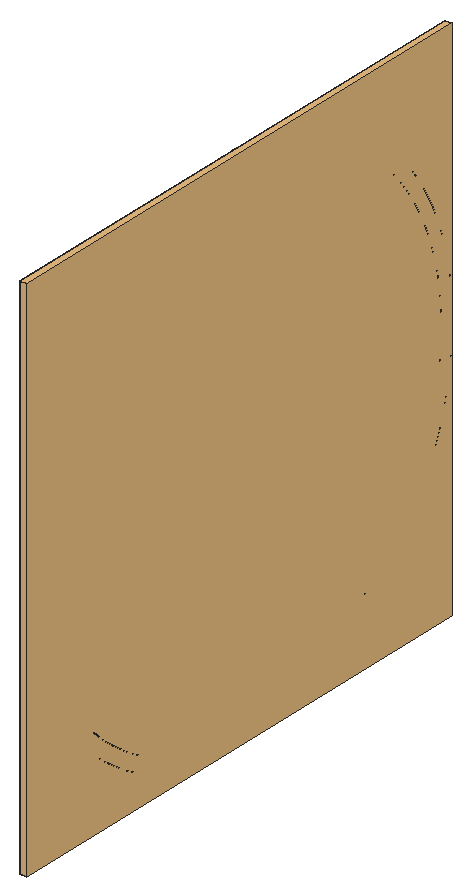
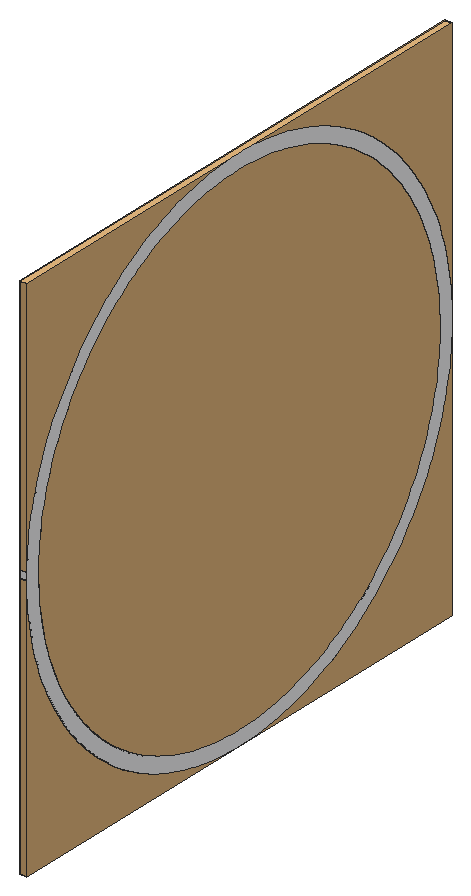
# SketchUp Ruby script. Lengths in inches.
U = 1.inch
M = Sketchup.active_model
def pt(a) = Geom::Point3d.new(a.map { |v| v * U })
def face(e, loops, mat)
  f = e.add_face(loops[0].map { |a| pt(a) })
  loops[1..].each { |l| e.add_face(l.map { |a| pt(a) }).erase! }
  f.material = f.back_material = mat if mat
  f
end
# faces: each face lists its corners as indices into pts; further lists are holes
def faces(e, pts, list, mat = nil) = list.each { |f| face(e, (f[0].is_a?(Array) ? f : [f]).map { |l| l.map { |i| pts[i] } }, mat) }
# xy, xz, yz: faces in a plane at the given z, y or x. An outline is a flat list of corners, or four numbers for a rectangle; further outlines are holes
def ring(l) = l.size == 4 ? [[l[0], l[1]], [l[2], l[1]], [l[2], l[3]], [l[0], l[3]]] : l.each_slice(2).to_a
def flat(e, list, mat, &to3) = list.each { |f| face(e, (f[0].is_a?(Array) ? f : [f]).map { |l| ring(l).map { |u, v| to3.(u, v) } }, mat) }
def xy(e, z, list, mat = nil) = flat(e, list, mat) { |x, y| [x, y, z] }
def xz(e, y, list, mat = nil) = flat(e, list, mat) { |x, z| [x, y, z] }
def yz(e, x, list, mat = nil) = flat(e, list, mat) { |y, z| [x, y, z] }
def lines(e, pts, list) = list.each { |a, b| e.add_line(pt(pts[a]), pt(pts[b])) }
# prism: a flat outline (further loops are holes) pulled along v
def prism(e, loops, v, mat = nil)
  f = face(e, loops, mat); d = Geom::Vector3d.new(v.map { |x| x * U })
  f.pushpull(f.normal.samedirection?(d) ? d.length : -d.length)
end
def box(e, o, s, mat = nil) = prism(e, [[o, [o[0] + s[0], o[1], o[2]], [o[0] + s[0], o[1] + s[1], o[2]], [o[0], o[1] + s[1], o[2]]]], [0, 0, s[2]], mat)
def at(x, y, z, deg = 0) = Geom::Transformation.translation(pt([x, y, z])) * Geom::Transformation.rotation(ORIGIN, Z_AXIS, deg.degrees)
def axes(o, x, y, z) = Geom::Transformation.new([*x, 0, *y, 0, *z, 0, *pt(o).to_a, 1])
def part(name) = M.definitions.add(name)
# library, detail: a bought-in or finely detailed component or shape, given as its bounding box
def library(name, o, s) = part(name).tap { |d| box(d.entities, o, s) }
def detail(e, o, s) = box(e.add_group.entities, o, s)
def put(e, d, t, mat = nil) = e.add_instance(d, t).tap { |i| i.material = mat if mat }
def group(e, t, mat = nil) = e.add_group.tap { |g| g.transformation = t; g.material = mat if mat }.entities
root = M.entities
M.materials.add("False Ceiling Light").color = [254, 227, 169]
M.materials.add("[Quartz Light Grey]").color = [251, 251, 252]
c1 = library("Group\#30",[0,0,0],[0.5,38,38])
xy(root,32,[[44.5,229.9375,45,230.44]],"[Quartz Light Grey]")
xy(root,33,[[44.5,229.94,45,230.41]],"[Quartz Light Grey]")
xz(root,248,[[44.5,50.94,45,51.41]],"[Quartz Light Grey]")
xz(root,249,[[44.5,50.9375,45,51.44]],"[Quartz Light Grey]")
yz(root,44.5,[[[229.9375,32,230.44,32,230.93,32.02,231.43,32.05,231.92,32.1,232.42,32.15,232.91,32.22,233.89,32.4,234.375,32.51,234.86,32.63,235.34,32.76,235.8125,32.91,236.28,33.07,236.75,33.24,237.21,33.42,237.67,33.62,238.125,33.82,238.57,34.04,239.01,34.27,239.45,34.51,240.3,35.03,241.12,35.59,241.52,35.89,241.91,36.2,242.29,36.51,242.67,36.84,243.39,37.52,243.74,37.875,244.08,38.24,244.41,38.61,244.73,38.99,245.04,39.38,245.33,39.78,245.625,40.1875,245.9,40.6,246.17,41.02,246.67,41.88,246.9,42.32,247.12,42.76,247.33,43.22,247.53,43.67,247.72,44.13,247.89,44.6,248.05,45.07,248.2,45.54,248.34,46.02,248.46,46.5,248.57,46.99,248.67,47.48,248.76,47.97,248.83,48.46,248.89,48.95,248.9375,49.45,248.97,49.94,248.99,50.44,249,50.9375,249,51.44,248.98,51.93,248.95,52.43,248.9,52.92,248.85,53.42,248.78,53.91,248.6,54.89,248.49,55.375,248.37,55.86,248.24,56.34,248.09,56.8125,247.93,57.28,247.76,57.75,247.58,58.21,247.38,58.67,247.18,59.125,246.96,59.57,246.73,60.01,246.49,60.45,245.97,61.3,245.41,62.12,245.11,62.52,244.8,62.91,244.49,63.29,244.16,63.67,243.48,64.39,243.125,64.74,242.76,65.08,242.39,65.41,242.01,65.73,241.62,66.04,241.22,66.33,240.8125,66.625,240.4,66.9,239.98,67.17,239.12,67.67,238.68,67.9,238.24,68.12,237.78,68.33,237.33,68.53,236.87,68.72,236.4,68.89,235.93,69.05,235.46,69.2,234.98,69.34,234.5,69.46,234.01,69.57,233.52,69.67,233.03,69.76,232.54,69.83,232.05,69.89,231.55,69.9375,231.06,69.97,230.56,69.99,230.0625,70,229.56,70,229.07,69.98,228.57,69.95,228.08,69.9,227.58,69.85,227.09,69.78,226.11,69.6,225.625,69.49,225.14,69.37,224.66,69.24,224.1875,69.09,223.72,68.93,223.25,68.76,222.79,68.58,222.33,68.38,221.875,68.18,221.43,67.96,220.99,67.73,220.55,67.49,219.7,66.97,218.88,66.41,218.48,66.11,218.09,65.8,217.71,65.49,217.33,65.16,216.61,64.48,216.26,64.125,215.92,63.76,215.59,63.39,215.27,63.01,214.96,62.62,214.67,62.22,214.375,61.8125,214.1,61.4,213.83,60.98,213.33,60.12,213.1,59.68,212.88,59.24,212.67,58.78,212.47,58.33,212.28,57.87,212.11,57.4,211.95,56.93,211.8,56.46,211.66,55.98,211.54,55.5,211.43,55.01,211.33,54.52,211.24,54.03,211.17,53.54,211.11,53.05,211.0625,52.55,211.03,52.06,211.01,51.56,211,51.0625,211,50.56,211.02,50.07,211.05,49.57,211.1,49.08,211.15,48.58,211.22,48.09,211.4,47.11,211.51,46.625,211.63,46.14,211.76,45.66,211.91,45.1875,212.07,44.72,212.24,44.25,212.42,43.79,212.62,43.33,212.82,42.875,213.04,42.43,213.27,41.99,213.51,41.55,214.03,40.7,214.59,39.88,214.89,39.48,215.2,39.09,215.51,38.71,215.84,38.33,216.52,37.61,216.875,37.26,217.24,36.92,217.61,36.59,217.99,36.27,218.38,35.96,218.78,35.67,219.1875,35.375,219.6,35.1,220.02,34.83,220.88,34.33,221.32,34.1,221.76,33.88,222.22,33.67,222.67,33.47,223.13,33.28,223.6,33.11,224.07,32.95,224.54,32.8,225.02,32.66,225.5,32.54,225.99,32.43,226.48,32.33,226.97,32.24,227.46,32.17,227.95,32.11,228.45,32.0625,228.94,32.03,229.44,32.01],[229.94,33,229.47,33.01,229,33.03,228.53,33.06,228.06,33.1,227.59,33.16,227.125,33.23,226.66,33.3125,226.2,33.41,225.74,33.51,225.28,33.63,224.83,33.76,224.38,33.9,223.9375,34.05,223.49,34.22,223.06,34.39,222.625,34.58,222.2,34.78,221.78,34.99,221.36,35.21,220.95,35.44,220.55,35.68,220.15,35.9375,219.76,36.2,219.37,36.47,219,36.76,218.625,37.05,218.27,37.35,217.91,37.66,217.57,37.98,217.23,38.3125,216.9,38.65,216.58,39,216.27,39.35,215.97,39.72,215.68,40.09,215.4,40.47,215.13,40.85,214.87,41.25,214.62,41.65,214.38,42.05,214.15,42.46,213.73,43.3,213.53,43.73,213.35,44.17,213.17,44.6,213.01,45.05,212.86,45.49,212.72,45.94,212.48,46.86,212.38,47.31,212.29,47.78,212.21,48.24,212.09,49.18,212.05,49.65,212.02,50.12,212,50.59,212,51.06,212.01,51.53,212.03,52,212.06,52.47,212.1,52.94,212.16,53.41,212.23,53.875,212.3125,54.34,212.41,54.8,212.51,55.26,212.63,55.72,212.76,56.17,212.9,56.62,213.05,57.0625,213.22,57.51,213.39,57.94,213.58,58.375,213.78,58.8,213.99,59.22,214.21,59.64,214.44,60.05,214.68,60.45,214.9375,60.85,215.2,61.24,215.47,61.63,215.76,62,216.05,62.375,216.35,62.73,216.66,63.09,216.98,63.43,217.3125,63.77,217.65,64.1,218,64.42,218.35,64.73,218.72,65.03,219.09,65.32,219.47,65.6,219.85,65.87,220.25,66.13,220.65,66.38,221.05,66.62,221.46,66.85,222.3,67.27,222.73,67.47,223.17,67.65,223.6,67.83,224.05,67.99,224.49,68.14,224.94,68.28,225.86,68.52,226.31,68.62,226.78,68.71,227.24,68.79,228.18,68.91,228.65,68.95,229.12,68.98,229.59,69,230.06,69,230.53,68.99,231,68.97,231.47,68.94,231.94,68.9,232.41,68.84,232.875,68.77,233.34,68.6875,233.8,68.59,234.26,68.49,234.72,68.37,235.17,68.24,235.62,68.1,236.0625,67.95,236.51,67.78,236.94,67.61,237.375,67.42,237.8,67.22,238.22,67.01,238.64,66.79,239.05,66.56,239.45,66.32,239.85,66.0625,240.24,65.8,240.63,65.53,241,65.24,241.375,64.95,241.73,64.65,242.09,64.34,242.43,64.02,242.77,63.6875,243.1,63.35,243.42,63,243.73,62.65,244.03,62.28,244.32,61.91,244.6,61.53,244.87,61.15,245.13,60.75,245.38,60.35,245.62,59.95,245.85,59.54,246.27,58.7,246.47,58.27,246.65,57.83,246.83,57.4,246.99,56.95,247.14,56.51,247.28,56.06,247.52,55.14,247.62,54.69,247.71,54.22,247.79,53.76,247.91,52.82,247.95,52.35,247.98,51.88,248,51.41,248,50.94,247.99,50.47,247.97,50,247.94,49.53,247.9,49.06,247.84,48.59,247.77,48.125,247.6875,47.66,247.59,47.2,247.49,46.74,247.37,46.28,247.24,45.83,247.1,45.38,246.95,44.9375,246.78,44.49,246.61,44.06,246.42,43.625,246.22,43.2,246.01,42.78,245.79,42.36,245.56,41.95,245.32,41.55,245.0625,41.15,244.8,40.76,244.53,40.37,244.24,40,243.95,39.625,243.65,39.27,243.34,38.91,243.02,38.57,242.6875,38.23,242.35,37.9,242,37.58,241.65,37.27,241.28,36.97,240.91,36.68,240.53,36.4,240.15,36.13,239.75,35.87,239.35,35.62,238.95,35.38,238.54,35.15,237.7,34.73,237.27,34.53,236.83,34.35,236.4,34.17,235.95,34.01,235.51,33.86,235.06,33.72,234.14,33.48,233.69,33.38,233.22,33.29,232.76,33.21,231.82,33.09,231.35,33.05,230.88,33.02,230.41,33]]],"[Quartz Light Grey]")
p = [[45,228.45,32.0625],[45,228.94,32.03],[44.5,228.94,32.03],[44.5,228.45,32.0625],[45,229.44,32.01],[44.5,229.44,32.01],
  [45,229.9375,32],[44.5,229.9375,32],[45,230.44,32],[45,230.93,32.02],[44.5,230.93,32.02],[44.5,230.44,32],
  [45,231.43,32.05],[44.5,231.43,32.05],[45,227.46,32.17],[45,227.95,32.11],[44.5,227.95,32.11],[44.5,227.46,32.17],
  [45,231.92,32.1],[44.5,231.92,32.1],[45,232.42,32.15],[44.5,232.42,32.15],[45,226.48,32.33],[45,226.97,32.24],
  [44.5,226.97,32.24],[44.5,226.48,32.33],[45,232.91,32.22],[44.5,232.91,32.22],[45,233.4,32.31],[44.5,233.4,32.31],
  [45,225.99,32.43],[44.5,225.99,32.43],[45,233.89,32.4],[44.5,233.89,32.4],[45,225.5,32.54],[44.5,225.5,32.54],
  [45,234.375,32.51],[44.5,234.375,32.51],[45,225.02,32.66],[44.5,225.02,32.66],[45,234.86,32.63],[44.5,234.86,32.63],
  [45,235.34,32.76],[44.5,235.34,32.76],[45,224.54,32.8],[44.5,224.54,32.8],[45,224.07,32.95],[44.5,224.07,32.95],
  [45,235.8125,32.91],[44.5,235.8125,32.91],[45,223.6,33.11],[44.5,223.6,33.11],[45,236.28,33.07],[44.5,236.28,33.07],
  [45,229,33.03],[45,228.53,33.06],[44.5,228.53,33.06],[44.5,229,33.03],[45,229.47,33.01],[44.5,229.47,33.01],
  [45,229.94,33],[44.5,229.94,33],[45,230.88,33.02],[45,230.41,33],[44.5,230.41,33],[44.5,230.88,33.02],
  [45,231.35,33.05],[44.5,231.35,33.05],[45,223.13,33.28],[44.5,223.13,33.28],[45,228.06,33.1],[45,227.59,33.16],
  [44.5,227.59,33.16],[44.5,228.06,33.1],[45,231.82,33.09],[44.5,231.82,33.09],[45,232.29,33.15],[44.5,232.29,33.15],
  [45,232.76,33.21],[44.5,232.76,33.21],[45,236.75,33.24],[44.5,236.75,33.24],[45,227.125,33.23],[45,226.66,33.3125],
  [44.5,226.66,33.3125],[44.5,227.125,33.23],[45,233.22,33.29],[44.5,233.22,33.29],[45,237.21,33.42],[44.5,237.21,33.42],
  [45,222.67,33.47],[44.5,222.67,33.47],[45,226.2,33.41],[44.5,226.2,33.41],[45,233.69,33.38],[44.5,233.69,33.38],
  [45,225.74,33.51],[44.5,225.74,33.51],[45,234.14,33.48],[44.5,234.14,33.48],[45,237.67,33.62],[44.5,237.67,33.62],
  [45,222.22,33.67],[44.5,222.22,33.67],[45,225.28,33.63],[44.5,225.28,33.63],[45,234.6,33.6],[44.5,234.6,33.6],
  [45,224.83,33.76],[44.5,224.83,33.76],[45,235.06,33.72],[44.5,235.06,33.72],[45,238.125,33.82],[44.5,238.125,33.82],
  [45,221.76,33.88],[44.5,221.76,33.88],[45,235.51,33.86],[44.5,235.51,33.86],[45,224.38,33.9],[44.5,224.38,33.9],
  [45,238.57,34.04],[44.5,238.57,34.04],[45,221.32,34.1],[44.5,221.32,34.1],[45,223.9375,34.05],[44.5,223.9375,34.05],
  [45,235.95,34.01],[44.5,235.95,34.01],[45,236.4,34.17],[44.5,236.4,34.17],[45,239.01,34.27],[44.5,239.01,34.27],
  [45,220.88,34.33],[44.5,220.88,34.33],[45,223.49,34.22],[44.5,223.49,34.22],[45,223.06,34.39],[44.5,223.06,34.39],
  [45,236.83,34.35],[44.5,236.83,34.35],[45,220.45,34.58],[44.5,220.45,34.58],[45,237.27,34.53],[44.5,237.27,34.53],
  [45,239.45,34.51],[44.5,239.45,34.51],[45,222.625,34.58],[44.5,222.625,34.58],[45,237.7,34.73],[44.5,237.7,34.73],
  [45,239.875,34.77],[44.5,239.875,34.77],[45,220.02,34.83],[44.5,220.02,34.83],[45,222.2,34.78],[44.5,222.2,34.78],
  [45,238.12,34.94],[44.5,238.12,34.94],[45,219.6,35.1],[44.5,219.6,35.1],[45,221.78,34.99],[44.5,221.78,34.99],
  [45,240.3,35.03],[44.5,240.3,35.03],[45,238.54,35.15],[44.5,238.54,35.15],[45,221.36,35.21],[44.5,221.36,35.21],
  [45,240.71,35.31],[44.5,240.71,35.31],[45,219.1875,35.375],[44.5,219.1875,35.375],[45,220.95,35.44],[44.5,220.95,35.44],
  [45,238.95,35.38],[44.5,238.95,35.38],[45,241.12,35.59],[44.5,241.12,35.59],[45,218.78,35.67],[44.5,218.78,35.67],
  [45,220.55,35.68],[44.5,220.55,35.68],[45,239.35,35.62],[44.5,239.35,35.62],[45,239.75,35.87],[44.5,239.75,35.87],
  [45,241.52,35.89],[44.5,241.52,35.89],[45,218.38,35.96],[44.5,218.38,35.96],[45,220.15,35.9375],[44.5,220.15,35.9375],
  [45,219.76,36.2],[44.5,219.76,36.2],[45,240.15,36.13],[44.5,240.15,36.13],[45,241.91,36.2],[44.5,241.91,36.2],
  [45,217.99,36.27],[44.5,217.99,36.27],[45,240.53,36.4],[44.5,240.53,36.4],[45,219.37,36.47],[44.5,219.37,36.47],
  [45,242.29,36.51],[44.5,242.29,36.51],[45,217.61,36.59],[44.5,217.61,36.59],[45,240.91,36.68],[44.5,240.91,36.68],
  [45,219,36.76],[44.5,219,36.76],[45,242.67,36.84],[44.5,242.67,36.84],[45,217.24,36.92],[44.5,217.24,36.92],
  [45,241.28,36.97],[44.5,241.28,36.97],[45,218.625,37.05],[44.5,218.625,37.05],[45,243.03,37.18],[44.5,243.03,37.18],
  [45,218.27,37.35],[44.5,218.27,37.35],[45,241.65,37.27],[44.5,241.65,37.27],[45,243.39,37.52],[44.5,243.39,37.52],
  [45,242,37.58],[44.5,242,37.58],[45,217.91,37.66],[44.5,217.91,37.66],[45,243.74,37.875],[44.5,243.74,37.875],
  [45,242.35,37.9],[44.5,242.35,37.9],[45,217.57,37.98],[44.5,217.57,37.98],[45,242.6875,38.23],[44.5,242.6875,38.23],
  [45,244.08,38.24],[44.5,244.08,38.24],[45,217.23,38.3125],[44.5,217.23,38.3125],[45,243.02,38.57],[44.5,243.02,38.57],
  [45,244.41,38.61],[44.5,244.41,38.61],[45,216.9,38.65],[44.5,216.9,38.65],[45,243.34,38.91],[44.5,243.34,38.91],
  [45,244.73,38.99],[44.5,244.73,38.99],[45,243.65,39.27],[44.5,243.65,39.27],[45,245.04,39.38],[44.5,245.04,39.38],
  [45,243.95,39.625],[44.5,243.95,39.625],[45,245.33,39.78],[44.5,245.33,39.78],[45,244.24,40],[44.5,244.24,40],
  [45,245.625,40.1875],[44.5,245.625,40.1875],[45,244.53,40.37],[44.5,244.53,40.37],[45,245.9,40.6],[44.5,245.9,40.6],
  [45,244.8,40.76],[44.5,244.8,40.76],[45,246.17,41.02],[44.5,246.17,41.02],[45,245.0625,41.15],[44.5,245.0625,41.15],
  [45,246.42,41.45],[44.5,246.42,41.45],[45,245.32,41.55],[44.5,245.32,41.55],[45,246.67,41.88],[44.5,246.67,41.88],
  [45,245.56,41.95],[44.5,245.56,41.95],[45,245.79,42.36],[44.5,245.79,42.36],[45,246.9,42.32],[44.5,246.9,42.32],
  [45,247.12,42.76],[44.5,247.12,42.76],[45,246.01,42.78],[44.5,246.01,42.78],[45,246.22,43.2],[44.5,246.22,43.2],
  [45,247.33,43.22],[44.5,247.33,43.22],[45,246.42,43.625],[44.5,246.42,43.625],[45,247.53,43.67],[44.5,247.53,43.67],
  [45,246.61,44.06],[44.5,246.61,44.06],[45,247.72,44.13],[44.5,247.72,44.13],[45,246.78,44.49],[44.5,246.78,44.49],
  [45,247.89,44.6],[44.5,247.89,44.6],[45,246.95,44.9375],[44.5,246.95,44.9375],[45,248.05,45.07],[44.5,248.05,45.07],
  [45,247.1,45.38],[44.5,247.1,45.38],[45,248.2,45.54],[44.5,248.2,45.54],[45,247.24,45.83],[44.5,247.24,45.83],
  [45,248.34,46.02],[44.5,248.34,46.02],[45,247.37,46.28],[44.5,247.37,46.28],[45,248.46,46.5],[44.5,248.46,46.5],
  [45,247.49,46.74],[44.5,247.49,46.74],[45,248.57,46.99],[44.5,248.57,46.99],[45,247.59,47.2],[44.5,247.59,47.2],
  [45,248.67,47.48],[44.5,248.67,47.48],[45,247.6875,47.66],[44.5,247.6875,47.66],[45,248.76,47.97],[44.5,248.76,47.97],
  [45,247.77,48.125],[44.5,247.77,48.125],[45,248.83,48.46],[44.5,248.83,48.46],[45,247.84,48.59],[44.5,247.84,48.59],
  [45,248.89,48.95],[44.5,248.89,48.95],[45,247.9,49.06],[44.5,247.9,49.06],[45,248.9375,49.45],[44.5,248.9375,49.45],
  [45,247.94,49.53],[44.5,247.94,49.53],[45,248.97,49.94],[44.5,248.97,49.94],[45,247.97,50],[44.5,247.97,50],
  [45,248.99,50.44],[44.5,248.99,50.44],[45,247.99,50.47],[44.5,247.99,50.47],[45,249,50.9375],[44.5,249,50.9375],
  [45,248,50.94],[44.5,248,50.94],[45,247.98,51.88],[45,248,51.41],[44.5,248,51.41],[44.5,247.98,51.88],
  [45,249,51.44],[45,248.98,51.93],[44.5,248.98,51.93],[44.5,249,51.44],[45,247.95,52.35],[44.5,247.95,52.35],
  [45,248.95,52.43],[44.5,248.95,52.43],[45,247.91,52.82],[44.5,247.91,52.82],[45,248.9,52.92],[44.5,248.9,52.92],
  [45,247.85,53.29],[44.5,247.85,53.29],[45,248.85,53.42],[44.5,248.85,53.42],[45,247.79,53.76],[44.5,247.79,53.76],
  [45,248.78,53.91],[44.5,248.78,53.91],[45,247.71,54.22],[44.5,247.71,54.22],[45,248.69,54.4],[44.5,248.69,54.4],
  [45,247.62,54.69],[44.5,247.62,54.69],[45,248.6,54.89],[44.5,248.6,54.89],[45,247.52,55.14],[44.5,247.52,55.14],
  [45,248.49,55.375],[44.5,248.49,55.375],[45,247.4,55.6],[44.5,247.4,55.6],[45,248.37,55.86],[44.5,248.37,55.86],
  [45,247.28,56.06],[44.5,247.28,56.06],[45,248.24,56.34],[44.5,248.24,56.34],[45,247.14,56.51],[44.5,247.14,56.51],
  [45,248.09,56.8125],[44.5,248.09,56.8125],[45,246.99,56.95],[44.5,246.99,56.95],[45,247.93,57.28],[44.5,247.93,57.28],
  [45,246.83,57.4],[44.5,246.83,57.4],[45,247.76,57.75],[44.5,247.76,57.75],[45,246.65,57.83],[44.5,246.65,57.83],
  [45,246.47,58.27],[44.5,246.47,58.27],[45,247.58,58.21],[44.5,247.58,58.21],[45,247.38,58.67],[44.5,247.38,58.67],
  [45,246.27,58.7],[44.5,246.27,58.7],[45,246.06,59.12],[44.5,246.06,59.12],[45,247.18,59.125],[44.5,247.18,59.125],
  [45,245.85,59.54],[44.5,245.85,59.54],[45,246.96,59.57],[44.5,246.96,59.57],[45,245.62,59.95],[44.5,245.62,59.95],
  [45,246.73,60.01],[44.5,246.73,60.01],[45,245.38,60.35],[44.5,245.38,60.35],[45,246.49,60.45],[44.5,246.49,60.45],
  [45,245.13,60.75],[44.5,245.13,60.75],[45,246.23,60.875],[44.5,246.23,60.875],[45,244.87,61.15],[44.5,244.87,61.15],
  [45,245.97,61.3],[44.5,245.97,61.3],[45,244.6,61.53],[44.5,244.6,61.53],[45,245.69,61.71],[44.5,245.69,61.71],
  [45,244.32,61.91],[44.5,244.32,61.91],[45,245.41,62.12],[44.5,245.41,62.12],[45,244.03,62.28],[44.5,244.03,62.28],
  [45,245.11,62.52],[44.5,245.11,62.52],[45,243.73,62.65],[44.5,243.73,62.65],[45,244.8,62.91],[44.5,244.8,62.91]]
faces(root,p,[[0,1,2,3],[1,4,5,2],[4,6,7,5],[8,9,10,11],[9,12,13,10],[14,15,16,17],[15,0,3,16],[12,18,19,13],
  [18,20,21,19],[22,23,24,25],[23,14,17,24],[20,26,27,21],[26,28,29,27],[30,22,25,31],[28,32,33,29],[34,30,31,35],
  [32,36,37,33],[38,34,35,39],[36,40,41,37],[40,42,43,41],[44,38,39,45],[46,44,45,47],[42,48,49,43],[50,46,47,51],
  [48,52,53,49],[54,55,56,57],[58,54,57,59],[60,58,59,61],[62,63,64,65],[66,62,65,67],[68,50,51,69],[70,71,72,73],
  [55,70,73,56],[74,66,67,75],[76,74,75,77],[78,76,77,79],[52,80,81,53],[82,83,84,85],[71,82,85,72],[86,78,79,87],
  [80,88,89,81],[90,68,69,91],[83,92,93,84],[94,86,87,95],[92,96,97,93],[98,94,95,99],[88,100,101,89],[102,90,91,103],
  [96,104,105,97],[106,98,99,107],[104,108,109,105],[110,106,107,111],[100,112,113,101],[114,102,103,115],[116,110,111,117],[108,118,119,109],
  [112,120,121,113],[122,114,115,123],[118,124,125,119],[126,116,117,127],[128,126,127,129],[120,130,131,121],[132,122,123,133],[124,134,135,125],
  [134,136,137,135],[138,128,129,139],[140,132,133,141],[142,138,139,143],[130,144,145,131],[136,146,147,137],[148,142,143,149],[144,150,151,145],
  [152,140,141,153],[146,154,155,147],[156,148,149,157],[158,152,153,159],[154,160,161,155],[150,162,163,151],[164,156,157,165],[160,166,167,161],
  [162,168,169,163],[170,158,159,171],[166,172,173,167],[174,164,165,175],[168,176,177,169],[178,170,171,179],[172,180,181,173],[182,174,175,183],
  [184,182,183,185],[176,186,187,177],[188,178,179,189],[180,190,191,181],[190,192,193,191],[194,184,185,195],[186,196,197,187],[198,188,189,199],
  [200,194,195,201],[192,202,203,193],[196,204,205,197],[206,198,199,207],[208,200,201,209],[202,210,211,203],[204,212,213,205],[214,206,207,215],
  [216,208,209,217],[210,218,219,211],[212,220,221,213],[218,222,223,219],[224,216,217,225],[220,226,227,221],[228,224,225,229],[222,230,231,223],
  [226,232,233,227],[234,228,229,235],[230,236,237,231],[238,234,235,239],[232,240,241,233],[236,242,243,237],[244,238,239,245],[240,246,247,241],
  [242,248,249,243],[250,244,245,251],[246,252,253,247],[254,250,251,255],[252,256,257,253],[258,254,255,259],[256,260,261,257],[262,258,259,263],
  [260,264,265,261],[266,262,263,267],[264,268,269,265],[270,266,267,271],[268,272,273,269],[274,270,271,275],[272,276,277,273],[278,274,275,279],
  [276,280,281,277],[282,278,279,283],[284,282,283,285],[280,286,287,281],[286,288,289,287],[290,284,285,291],[292,290,291,293],[288,294,295,289],
  [296,292,293,297],[294,298,299,295],[300,296,297,301],[298,302,303,299],[304,300,301,305],[302,306,307,303],[308,304,305,309],[306,310,311,307],
  [312,308,309,313],[310,314,315,311],[316,312,313,317],[314,318,319,315],[320,316,317,321],[318,322,323,319],[324,320,321,325],[322,326,327,323],
  [328,324,325,329],[326,330,331,327],[332,328,329,333],[330,334,335,331],[336,332,333,337],[334,338,339,335],[340,336,337,341],[338,342,343,339],
  [344,340,341,345],[342,346,347,343],[348,344,345,349],[346,350,351,347],[352,348,349,353],[350,354,355,351],[356,352,353,357],[354,358,359,355],
  [360,356,357,361],[362,363,364,365],[366,367,368,369],[370,362,365,371],[367,372,373,368],[374,370,371,375],[372,376,377,373],[378,374,375,379],
  [376,380,381,377],[382,378,379,383],[380,384,385,381],[386,382,383,387],[384,388,389,385],[390,386,387,391],[388,392,393,389],[394,390,391,395],
  [392,396,397,393],[398,394,395,399],[396,400,401,397],[402,398,399,403],[400,404,405,401],[406,402,403,407],[404,408,409,405],[410,406,407,411],
  [408,412,413,409],[414,410,411,415],[412,416,417,413],[418,414,415,419],[420,418,419,421],[416,422,423,417],[422,424,425,423],[426,420,421,427],
  [428,426,427,429],[424,430,431,425],[432,428,429,433],[430,434,435,431],[436,432,433,437],[434,438,439,435],[440,436,437,441],[438,442,443,439],
  [444,440,441,445],[442,446,447,443],[448,444,445,449],[446,450,451,447],[452,448,449,453],[450,454,455,451],[456,452,453,457],[454,458,459,455],
  [460,456,457,461],[458,462,463,459],[464,460,461,465],[462,466,467,463]],"[Quartz Light Grey]")
put(root,c1,at(44.5,211,32),"False Ceiling Light")
